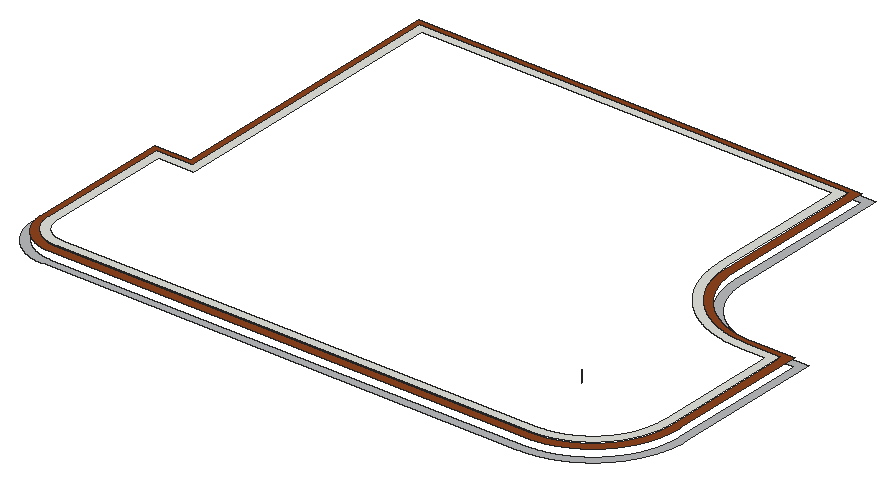
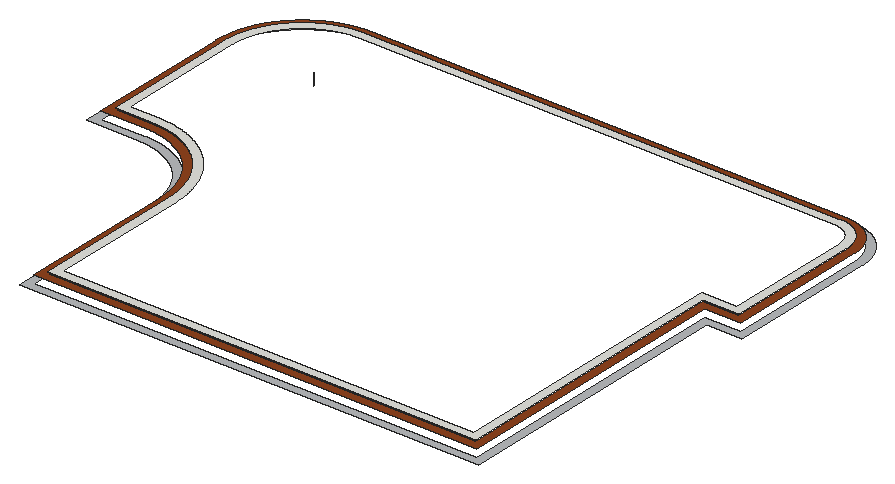
# SketchUp Ruby script. Lengths in inches.
U = 1.inch
M = Sketchup.active_model
def pt(a) = Geom::Point3d.new(a.map { |v| v * U })
def face(e, loops, mat)
  f = e.add_face(loops[0].map { |a| pt(a) })
  loops[1..].each { |l| e.add_face(l.map { |a| pt(a) }).erase! }
  f.material = f.back_material = mat if mat
  f
end
# faces: each face lists its corners as indices into pts; further lists are holes
def faces(e, pts, list, mat = nil) = list.each { |f| face(e, (f[0].is_a?(Array) ? f : [f]).map { |l| l.map { |i| pts[i] } }, mat) }
# xy, xz, yz: faces in a plane at the given z, y or x. An outline is a flat list of corners, or four numbers for a rectangle; further outlines are holes
def ring(l) = l.size == 4 ? [[l[0], l[1]], [l[2], l[1]], [l[2], l[3]], [l[0], l[3]]] : l.each_slice(2).to_a
def flat(e, list, mat, &to3) = list.each { |f| face(e, (f[0].is_a?(Array) ? f : [f]).map { |l| ring(l).map { |u, v| to3.(u, v) } }, mat) }
def xy(e, z, list, mat = nil) = flat(e, list, mat) { |x, y| [x, y, z] }
def xz(e, y, list, mat = nil) = flat(e, list, mat) { |x, z| [x, y, z] }
def yz(e, x, list, mat = nil) = flat(e, list, mat) { |y, z| [x, y, z] }
def lines(e, pts, list) = list.each { |a, b| e.add_line(pt(pts[a]), pt(pts[b])) }
# prism: a flat outline (further loops are holes) pulled along v
def prism(e, loops, v, mat = nil)
  f = face(e, loops, mat); d = Geom::Vector3d.new(v.map { |x| x * U })
  f.pushpull(f.normal.samedirection?(d) ? d.length : -d.length)
end
def box(e, o, s, mat = nil) = prism(e, [[o, [o[0] + s[0], o[1], o[2]], [o[0] + s[0], o[1] + s[1], o[2]], [o[0], o[1] + s[1], o[2]]]], [0, 0, s[2]], mat)
def at(x, y, z, deg = 0) = Geom::Transformation.translation(pt([x, y, z])) * Geom::Transformation.rotation(ORIGIN, Z_AXIS, deg.degrees)
def axes(o, x, y, z) = Geom::Transformation.new([*x, 0, *y, 0, *z, 0, *pt(o).to_a, 1])
def part(name) = M.definitions.add(name)
# library, detail: a bought-in or finely detailed component or shape, given as its bounding box
def library(name, o, s) = part(name).tap { |d| box(d.entities, o, s) }
def detail(e, o, s) = box(e.add_group.entities, o, s)
def put(e, d, t, mat = nil) = e.add_instance(d, t).tap { |i| i.material = mat if mat }
def group(e, t, mat = nil) = e.add_group.tap { |g| g.transformation = t; g.material = mat if mat }.entities
root = M.entities
M.materials.add("1427 AP 686 ARMOUR-N").color = [184, 186, 189]
M.materials.add("[Wood Fence]").color = [142, 67, 30]
xy(root,240,[[[20.991,129.924,20.843,129.925,20.686,129.928,20.529,129.934,20.372,129.941,20.215,129.95,20.059,129.961,19.902,129.975,19.746,129.99,19.59,130.008,19.434,130.027,19.278,130.049,19.123,130.072,18.968,130.098,18.813,130.125,18.659,130.155,18.505,130.187,18.352,130.22,18.199,130.256,18.046,130.294,17.894,130.333,17.743,130.375,17.592,130.419,17.442,130.464,17.292,130.512,17.143,130.561,16.994,130.613,16.847,130.666,16.7,130.721,16.553,130.779,16.408,130.838,16.263,130.899,16.119,130.962,15.976,131.027,15.834,131.093,15.693,131.162,15.552,131.232,15.413,131.305,15.274,131.379,15.137,131.454,15,131.532,14.865,131.611,14.73,131.693,14.597,131.776,14.464,131.86,14.333,131.947,14.203,132.035,14.074,132.125,13.947,132.216,13.82,132.309,13.695,132.404,13.571,132.501,13.448,132.599,13.327,132.698,13.207,132.799,13.088,132.902,12.854,133.112,12.74,133.22,12.627,133.329,12.515,133.439,12.404,133.551,12.296,133.664,12.188,133.779,12.082,133.895,11.978,134.012,11.875,134.131,11.774,134.251,11.674,134.373,11.576,134.495,11.48,134.619,11.385,134.744,11.292,134.871,11.2,134.999,11.111,135.127,11.022,135.258,10.936,135.389,10.851,135.521,10.768,135.654,10.687,135.789,10.608,135.924,10.53,136.061,10.454,136.198,10.38,136.337,10.308,136.476,10.238,136.617,10.169,136.758,10.102,136.9,10.038,137.044,9.975,137.1875,9.914,137.332,9.854,137.478,9.797,137.624,9.742,137.771,9.688,137.919,9.637,138.067,9.587,138.216,9.54,138.366,9.494,138.516,9.451,138.667,9.409,138.819,9.369,138.971,9.332,139.123,9.296,139.276,9.262,139.429,9.231,139.583,9.201,139.738,9.173,139.892,9.148,140.047,9.124,140.202,9.103,140.358,9.083,140.514,9.066,140.67,9.05,140.826,9.037,140.983,9.026,141.14,9.017,141.296,9.009,141.453,9.004,141.61,9.001,141.767,9,141.924,9,180,18,180,18,252,134,252,134,209.973,134.001,209.783,134.005,209.565,134.012,209.348,134.021,209.13,134.033,208.913,134.047,208.696,134.064,208.479,134.084,208.263,134.106,208.046,134.131,207.83,134.159,207.615,134.189,207.399,134.221,207.184,134.257,206.97,134.295,206.755,134.335,206.542,134.378,206.329,134.424,206.116,134.472,205.904,134.523,205.692,134.576,205.481,134.632,205.271,134.69,205.062,134.751,204.853,134.815,204.645,134.881,204.4375,134.949,204.231,135.02,204.026,135.094,203.821,135.17,203.617,135.248,203.414,135.329,203.212,135.412,203.011,135.498,202.811,135.586,202.613,135.676,202.415,135.769,202.218,135.864,202.022,135.962,201.828,136.062,201.635,136.164,201.443,136.268,201.252,136.375,201.063,136.484,200.875,136.596,200.688,136.709,200.502,136.825,200.318,136.943,200.136,137.064,199.954,137.186,199.775,137.311,199.596,137.4375,199.42,137.566,199.245,137.697,199.071,137.831,198.899,137.966,198.729,138.103,198.56,138.242,198.393,138.383,198.227,138.527,198.064,138.672,197.902,138.819,197.742,138.968,197.583,139.119,197.427,139.272,197.272,139.427,197.119,139.583,196.968,139.742,196.819,139.902,196.672,140.064,196.527,140.227,196.383,140.393,196.242,140.56,196.103,140.729,195.966,140.899,195.831,141.071,195.697,141.245,195.566,141.42,195.4375,141.596,195.311,141.775,195.186,141.954,195.064,142.136,194.943,142.318,194.825,142.502,194.709,142.688,194.596,142.875,194.484,143.063,194.375,143.252,194.268,143.443,194.164,143.635,194.062,143.828,193.962,144.022,193.864,144.218,193.769,144.415,193.676,144.613,193.586,144.811,193.498,145.011,193.412,145.212,193.329,145.414,193.248,145.617,193.17,145.821,193.094,146.026,193.02,146.231,192.949,146.4375,192.881,146.645,192.815,146.853,192.751,147.062,192.69,147.271,192.632,147.481,192.576,147.692,192.523,147.904,192.472,148.116,192.424,148.329,192.378,148.542,192.335,148.755,192.295,148.97,192.257,149.184,192.221,149.399,192.189,149.615,192.159,149.83,192.131,150.046,192.106,150.263,192.084,150.479,192.064,150.696,192.047,150.913,192.033,151.13,192.021,151.348,192.012,151.565,192.005,151.783,192.001,151.973,192,165,192,165,153.924,164.998,153.634,164.993,153.344,164.984,153.055,164.972,152.765,164.956,152.475,164.937,152.186,164.914,151.897,164.888,151.608,164.858,151.32,164.825,151.031,164.788,150.744,164.748,150.457,164.704,150.17,164.657,149.884,164.607,149.598,164.553,149.313,164.495,149.029,164.434,148.745,164.37,148.463,164.302,148.181,164.231,147.9,164.157,147.619,164.079,147.34,163.997,147.062,163.913,146.784,163.825,146.508,163.734,146.233,163.639,145.958,163.541,145.686,163.44,145.414,163.335,145.143,163.228,144.874,163.117,144.606,163.002,144.34,162.885,144.074,162.764,143.811,162.641,143.548,162.514,143.288,162.383,143.028,162.25,142.771,162.114,142.515,161.974,142.261,161.832,142.008,161.687,141.757,161.538,141.508,161.386,141.261,161.232,141.015,161.074,140.772,160.914,140.53,160.751,140.291,160.585,140.053,160.416,139.817,160.244,139.584,160.069,139.352,159.891,139.123,159.711,138.896,159.528,138.671,159.343,138.448,159.154,138.228,158.963,138.009,158.77,137.793,158.573,137.58,158.375,137.369,158.173,137.16,157.97,136.954,157.763,136.75,157.554,136.549,157.343,136.35,157.13,136.154,156.914,135.96,156.696,135.769,156.475,135.581,156.252,135.395,156.027,135.212,155.8,135.032,155.571,134.854,155.339,134.68,155.106,134.508,154.87,134.339,154.632,134.173,154.393,134.009,154.151,133.849,153.908,133.692,153.662,133.537,153.415,133.386,153.166,133.237,152.915,133.092,152.662,132.949,152.408,132.81,152.152,132.673,151.894,132.54,151.635,132.41,151.375,132.283,151.112,132.159,150.849,132.039,150.583,131.921,150.317,131.807,150.049,131.696,149.78,131.588,149.509,131.484,149.237,131.383,148.964,131.285,148.69,131.19,148.415,131.099,148.139,131.011,147.861,130.926,147.583,130.845,147.304,130.767,147.023,130.693,146.742,130.622,146.46,130.554,146.177,130.49,145.894,130.429,145.61,130.372,145.325,130.318,145.039,130.267,144.753,130.22,144.466,130.176,144.179,130.136,143.891,130.099,143.603,130.066,143.315,130.036,143.026,130.01,142.737,129.987,142.447,129.968,142.158,129.952,141.868,129.94,141.578,129.931,141.288,129.926,141.003,129.924],[21.005,131.924,140.992,131.924,141.264,131.926,141.53,131.931,141.796,131.939,142.061,131.95,142.327,131.965,142.592,131.982,142.857,132.003,143.122,132.027,143.386,132.054,143.65,132.085,143.914,132.118,144.177,132.155,144.44,132.195,144.702,132.238,144.964,132.285,145.225,132.334,145.486,132.387,145.746,132.443,146.005,132.502,146.263,132.564,146.521,132.629,146.778,132.697,147.034,132.769,147.289,132.843,147.544,132.921,147.797,133.001,148.049,133.085,148.301,133.172,148.551,133.261,148.8,133.354,149.048,133.45,149.295,133.549,149.54,133.65,149.785,133.755,150.028,133.863,150.269,133.973,150.51,134.087,150.749,134.203,150.986,134.322,151.223,134.444,151.457,134.569,151.69,134.697,151.922,134.828,152.152,134.961,152.38,135.097,152.607,135.236,152.832,135.378,153.055,135.522,153.277,135.669,153.496,135.819,153.714,135.971,153.93,136.126,154.144,136.284,154.356,136.444,154.567,136.606,154.775,136.772,154.981,136.939,155.185,137.109,155.388,137.282,155.588,137.457,155.786,137.635,155.981,137.814,156.175,137.997,156.366,138.181,156.555,138.368,156.742,138.557,156.927,138.748,157.109,138.942,157.289,139.138,157.466,139.336,157.641,139.536,157.814,139.738,157.984,139.942,158.152,140.148,158.317,140.357,158.48,140.567,158.64,140.779,158.798,140.993,158.952,141.209,159.105,141.427,159.255,141.647,159.402,141.868,159.546,142.091,159.6875,142.316,159.826,142.543,159.963,142.771,160.096,143.001,160.227,143.233,160.354,143.466,160.479,143.7,160.601,143.937,160.721,144.174,160.837,144.413,160.951,144.654,161.061,144.895,161.169,145.138,161.274,145.383,161.375,145.628,161.474,145.875,161.57,146.123,161.663,146.372,161.752,146.622,161.839,146.874,161.923,147.126,162.003,147.379,162.081,147.634,162.155,147.889,162.227,148.145,162.295,148.402,162.36,148.659,162.422,148.918,162.481,149.177,162.537,149.437,162.59,149.698,162.639,149.959,162.686,150.221,162.729,150.483,162.769,150.746,162.806,151.009,162.839,151.273,162.87,151.537,162.897,151.801,162.921,152.066,162.942,152.331,162.96,152.596,162.974,152.862,162.985,153.127,162.994,153.393,162.998,153.659,163,153.931,163,190,151.967,190,151.758,190.001,151.517,190.006,151.275,190.013,151.034,190.023,150.792,190.036,150.551,190.052,150.31,190.071,150.07,190.093,149.829,190.118,149.589,190.146,149.35,190.176,149.11,190.21,148.871,190.246,148.633,190.285,148.395,190.327,148.157,190.372,147.921,190.42,147.684,190.471,147.449,190.525,147.214,190.581,146.979,190.64,146.746,190.702,146.513,190.767,146.281,190.835,146.05,190.905,145.82,190.979,145.59,191.055,145.362,191.134,145.134,191.215,144.908,191.299,144.682,191.387,144.458,191.476,144.235,191.569,144.013,191.664,143.792,191.762,143.572,191.862,143.353,191.965,143.136,192.071,142.92,192.18,142.705,192.291,142.492,192.404,142.28,192.52,142.07,192.639,141.861,192.76,141.653,192.884,141.447,193.01,141.243,193.139,141.04,193.27,140.838,193.404,140.639,193.54,140.441,193.679,140.244,193.819,140.05,193.963,139.857,194.108,139.665,194.256,139.476,194.406,139.289,194.559,139.103,194.714,138.919,194.87,138.737,195.03,138.557,195.191,138.38,195.354,138.204,195.52,138.03,195.688,137.858,195.858,137.688,196.03,137.52,196.204,137.354,196.38,137.191,196.557,137.03,196.737,136.87,196.919,136.714,197.103,136.559,197.289,136.406,197.476,136.256,197.665,136.108,197.857,135.963,198.05,135.819,198.244,135.679,198.441,135.54,198.639,135.404,198.838,135.27,199.04,135.139,199.243,135.01,199.447,134.884,199.653,134.76,199.861,134.639,200.07,134.52,200.28,134.404,200.492,134.291,200.705,134.18,200.92,134.071,201.136,133.965,201.353,133.862,201.572,133.762,201.792,133.664,202.013,133.569,202.235,133.476,202.458,133.387,202.682,133.299,202.908,133.215,203.134,133.134,203.362,133.055,203.59,132.979,203.82,132.905,204.05,132.835,204.281,132.767,204.513,132.702,204.746,132.64,204.979,132.581,205.214,132.525,205.449,132.471,205.684,132.42,205.921,132.372,206.157,132.327,206.395,132.285,206.633,132.246,206.871,132.21,207.11,132.176,207.35,132.146,207.589,132.118,207.829,132.093,208.07,132.071,208.31,132.052,208.551,132.036,208.792,132.023,209.034,132.013,209.275,132.006,209.517,132.001,209.758,132,209.967,132,250,20,250,20,178,11,178,11,141.931,11.001,141.793,11.004,141.663,11.008,141.532,11.014,141.401,11.022,141.27,11.031,141.14,11.042,141.009,11.055,140.879,11.069,140.749,11.086,140.619,11.104,140.489,11.123,140.36,11.145,140.231,11.168,140.102,11.192,139.973,11.219,139.845,11.247,139.717,11.276,139.59,11.308,139.463,11.341,139.336,11.376,139.21,11.412,139.084,11.45,138.959,11.49,138.834,11.531,138.71,11.574,138.586,11.618,138.463,11.664,138.341,11.712,138.219,11.761,138.098,11.812,137.977,11.865,137.857,11.919,137.738,11.974,137.619,12.031,137.501,12.09,137.384,12.15,137.268,12.212,137.153,12.275,137.038,12.34,136.924,12.406,136.811,12.474,136.699,12.543,136.588,12.613,136.478,12.685,136.369,12.759,136.26,12.834,136.153,12.91,136.047,12.988,135.941,13.067,135.837,13.147,135.733,13.229,135.631,13.312,135.53,13.396,135.43,13.482,135.331,13.569,135.233,13.657,135.136,13.746,135.041,13.837,134.946,13.929,134.853,14.022,134.761,14.212,134.581,14.309,134.493,14.407,134.406,14.506,134.32,14.606,134.236,14.707,134.153,14.809,134.071,14.913,133.991,15.017,133.912,15.122,133.834,15.229,133.758,15.336,133.683,15.444,133.61,15.554,133.538,15.664,133.467,15.775,133.398,15.887,133.33,16,133.264,16.114,133.199,16.229,133.136,16.344,133.075,16.46,133.014,16.577,132.956,16.695,132.899,16.814,132.843,16.933,132.789,17.053,132.736,17.173,132.686,17.295,132.636,17.416,132.589,17.539,132.542,17.662,132.498,17.786,132.455,17.91,132.414,18.035,132.374,18.16,132.336,18.286,132.3,18.412,132.265,18.539,132.232,18.666,132.201,18.793,132.171,18.921,132.143,19.049,132.117,19.178,132.092,19.307,132.069,19.436,132.048,19.565,132.028,19.695,132.01,19.825,131.994,19.955,131.979,20.085,131.966,20.216,131.955,20.346,131.946,20.477,131.938,20.607,131.932,20.738,131.928,20.869,131.925]]],"1427 AP 686 ARMOUR-N")
xy(root,242,[[[21.005,131.924,20.869,131.925,20.738,131.928,20.607,131.932,20.477,131.938,20.346,131.946,20.216,131.955,20.085,131.966,19.955,131.979,19.825,131.994,19.695,132.01,19.565,132.028,19.436,132.048,19.307,132.069,19.178,132.092,19.049,132.117,18.921,132.143,18.793,132.171,18.666,132.201,18.539,132.232,18.412,132.265,18.286,132.3,18.16,132.336,18.035,132.374,17.91,132.414,17.786,132.455,17.662,132.498,17.539,132.542,17.416,132.589,17.295,132.636,17.173,132.686,17.053,132.736,16.933,132.789,16.814,132.843,16.695,132.899,16.577,132.956,16.46,133.014,16.344,133.075,16.229,133.136,16.114,133.199,16,133.264,15.887,133.33,15.775,133.398,15.664,133.467,15.554,133.538,15.444,133.61,15.336,133.683,15.229,133.758,15.122,133.834,15.017,133.912,14.913,133.991,14.809,134.071,14.707,134.153,14.606,134.236,14.506,134.32,14.407,134.406,14.309,134.493,14.212,134.581,14.022,134.761,13.929,134.853,13.837,134.946,13.746,135.041,13.657,135.136,13.569,135.233,13.482,135.331,13.396,135.43,13.312,135.53,13.229,135.631,13.147,135.733,13.067,135.837,12.988,135.941,12.91,136.047,12.834,136.153,12.759,136.26,12.685,136.369,12.613,136.478,12.543,136.588,12.474,136.699,12.406,136.811,12.34,136.924,12.275,137.038,12.212,137.153,12.15,137.268,12.09,137.384,12.031,137.501,11.974,137.619,11.919,137.738,11.865,137.857,11.812,137.977,11.761,138.098,11.712,138.219,11.664,138.341,11.618,138.463,11.574,138.586,11.531,138.71,11.49,138.834,11.45,138.959,11.412,139.084,11.376,139.21,11.341,139.336,11.308,139.463,11.276,139.59,11.247,139.717,11.219,139.845,11.192,139.973,11.168,140.102,11.145,140.231,11.123,140.36,11.104,140.489,11.086,140.619,11.069,140.749,11.055,140.879,11.042,141.009,11.031,141.14,11.022,141.27,11.014,141.401,11.008,141.532,11.004,141.663,11.001,141.793,11,141.931,11,178,20,178,20,250,132,250,132,209.967,132.001,209.758,132.006,209.517,132.013,209.275,132.023,209.034,132.036,208.792,132.052,208.551,132.071,208.31,132.093,208.07,132.118,207.829,132.146,207.589,132.176,207.35,132.21,207.11,132.246,206.871,132.285,206.633,132.327,206.395,132.372,206.157,132.42,205.921,132.471,205.684,132.525,205.449,132.581,205.214,132.64,204.979,132.702,204.746,132.767,204.513,132.835,204.281,132.905,204.05,132.979,203.82,133.055,203.59,133.134,203.362,133.215,203.134,133.299,202.908,133.387,202.682,133.476,202.458,133.569,202.235,133.664,202.013,133.762,201.792,133.862,201.572,133.965,201.353,134.071,201.136,134.18,200.92,134.291,200.705,134.404,200.492,134.52,200.28,134.639,200.07,134.76,199.861,134.884,199.653,135.01,199.447,135.139,199.243,135.27,199.04,135.404,198.838,135.54,198.639,135.679,198.441,135.819,198.244,135.963,198.05,136.108,197.857,136.256,197.665,136.406,197.476,136.559,197.289,136.714,197.103,136.87,196.919,137.03,196.737,137.191,196.557,137.354,196.38,137.52,196.204,137.688,196.03,137.858,195.858,138.03,195.688,138.204,195.52,138.38,195.354,138.557,195.191,138.737,195.03,138.919,194.87,139.103,194.714,139.289,194.559,139.476,194.406,139.665,194.256,139.857,194.108,140.05,193.963,140.244,193.819,140.441,193.679,140.639,193.54,140.838,193.404,141.04,193.27,141.243,193.139,141.447,193.01,141.653,192.884,141.861,192.76,142.07,192.639,142.28,192.52,142.492,192.404,142.705,192.291,142.92,192.18,143.136,192.071,143.353,191.965,143.572,191.862,143.792,191.762,144.013,191.664,144.235,191.569,144.458,191.476,144.682,191.387,144.908,191.299,145.134,191.215,145.362,191.134,145.59,191.055,145.82,190.979,146.05,190.905,146.281,190.835,146.513,190.767,146.746,190.702,146.979,190.64,147.214,190.581,147.449,190.525,147.684,190.471,147.921,190.42,148.157,190.372,148.395,190.327,148.633,190.285,148.871,190.246,149.11,190.21,149.35,190.176,149.589,190.146,149.829,190.118,150.07,190.093,150.31,190.071,150.551,190.052,150.792,190.036,151.034,190.023,151.275,190.013,151.517,190.006,151.758,190.001,151.967,190,163,190,163,153.931,162.998,153.659,162.994,153.393,162.985,153.127,162.974,152.862,162.96,152.596,162.942,152.331,162.921,152.066,162.897,151.801,162.87,151.537,162.839,151.273,162.806,151.009,162.769,150.746,162.729,150.483,162.686,150.221,162.639,149.959,162.59,149.698,162.537,149.437,162.481,149.177,162.422,148.918,162.36,148.659,162.295,148.402,162.227,148.145,162.155,147.889,162.081,147.634,162.003,147.379,161.923,147.126,161.839,146.874,161.752,146.622,161.663,146.372,161.57,146.123,161.474,145.875,161.375,145.628,161.274,145.383,161.169,145.138,161.061,144.895,160.951,144.654,160.837,144.413,160.721,144.174,160.601,143.937,160.479,143.7,160.354,143.466,160.227,143.233,160.096,143.001,159.963,142.771,159.826,142.543,159.6875,142.316,159.546,142.091,159.402,141.868,159.255,141.647,159.105,141.427,158.952,141.209,158.798,140.993,158.64,140.779,158.48,140.567,158.317,140.357,158.152,140.148,157.984,139.942,157.814,139.738,157.641,139.536,157.466,139.336,157.289,139.138,157.109,138.942,156.927,138.748,156.742,138.557,156.555,138.368,156.366,138.181,156.175,137.997,155.981,137.814,155.786,137.635,155.588,137.457,155.388,137.282,155.185,137.109,154.981,136.939,154.775,136.772,154.567,136.606,154.356,136.444,154.144,136.284,153.93,136.126,153.714,135.971,153.496,135.819,153.277,135.669,153.055,135.522,152.832,135.378,152.607,135.236,152.38,135.097,152.152,134.961,151.922,134.828,151.69,134.697,151.457,134.569,151.223,134.444,150.986,134.322,150.749,134.203,150.51,134.087,150.269,133.973,150.028,133.863,149.785,133.755,149.54,133.65,149.295,133.549,149.048,133.45,148.8,133.354,148.551,133.261,148.301,133.172,148.049,133.085,147.797,133.001,147.544,132.921,147.289,132.843,147.034,132.769,146.778,132.697,146.521,132.629,146.263,132.564,146.005,132.502,145.746,132.443,145.486,132.387,145.225,132.334,144.964,132.285,144.702,132.238,144.44,132.195,144.177,132.155,143.914,132.118,143.65,132.085,143.386,132.054,143.122,132.027,142.857,132.003,142.592,131.982,142.327,131.965,142.061,131.95,141.796,131.939,141.53,131.931,141.264,131.926,140.992,131.924],[21.013,133.924,140.986,133.924,141.24,133.926,141.482,133.93,141.723,133.9375,141.965,133.948,142.206,133.961,142.447,133.977,142.688,133.996,142.929,134.018,143.169,134.043,143.409,134.07,143.649,134.101,143.888,134.134,144.127,134.171,144.366,134.21,144.604,134.252,144.841,134.297,145.078,134.345,145.314,134.396,145.55,134.449,145.785,134.506,146.019,134.565,146.253,134.627,146.485,134.692,146.717,134.76,146.949,134.83,147.179,134.903,147.408,134.979,147.637,135.058,147.864,135.14,148.091,135.224,148.316,135.311,148.541,135.401,148.764,135.493,148.986,135.589,149.207,135.686,149.427,135.787,149.645,135.89,149.863,135.996,150.079,136.104,150.293,136.215,150.506,136.329,150.718,136.445,150.929,136.564,151.138,136.685,151.346,136.809,151.552,136.935,151.756,137.064,151.959,137.195,152.16,137.329,152.36,137.465,152.558,137.603,152.755,137.744,152.949,137.887,153.142,138.033,153.333,138.181,153.523,138.331,153.71,138.483,153.896,138.638,154.08,138.795,154.261,138.954,154.441,139.116,154.619,139.279,154.795,139.445,154.969,139.612,155.141,139.782,155.311,139.954,155.479,140.128,155.644,140.304,155.808,140.482,155.969,140.662,156.128,140.844,156.285,141.028,156.44,141.213,156.593,141.401,156.743,141.59,156.891,141.781,157.036,141.974,157.179,142.169,157.32,142.365,157.459,142.563,157.595,142.763,157.729,142.964,157.86,143.167,157.989,143.372,158.115,143.578,158.239,143.785,158.36,143.994,158.479,144.205,158.595,144.417,158.708,144.63,158.819,144.845,158.928,145.061,159.034,145.278,159.137,145.496,159.237,145.716,159.335,145.937,159.43,146.159,159.523,146.383,159.613,146.607,159.7,146.832,159.784,147.059,159.866,147.286,159.945,147.515,160.021,147.744,160.094,147.974,160.164,148.206,160.232,148.4375,160.297,148.67,160.359,148.904,160.418,149.138,160.475,149.373,160.528,149.609,160.579,149.845,160.627,150.082,160.672,150.319,160.714,150.557,160.753,150.796,160.79,151.035,160.823,151.274,160.854,151.514,160.882,151.754,160.906,151.994,160.928,152.235,160.947,152.476,160.963,152.717,160.977,152.958,160.987,153.2,160.994,153.441,160.998,153.683,161,153.937,161,188,151.961,188,151.734,188.001,151.468,188.006,151.203,188.014,150.937,188.025,150.672,188.04,150.406,188.058,150.141,188.078,149.877,188.102,149.612,188.13,149.348,188.16,149.084,188.194,148.821,188.231,148.558,188.271,148.296,188.314,148.034,188.36,147.773,188.41,147.513,188.462,147.253,188.518,146.993,188.577,146.735,188.639,146.477,188.704,146.22,188.773,145.964,188.844,145.709,188.918,145.455,188.996,145.202,189.077,144.949,189.16,144.698,189.247,144.448,189.337,144.199,189.429,143.951,189.525,143.704,189.624,143.458,189.726,143.214,189.83,142.971,189.938,142.729,190.049,142.489,190.162,142.25,190.278,142.012,190.398,141.776,190.52,141.541,190.645,141.308,190.772,141.077,190.903,140.847,191.036,140.618,191.173,140.392,191.312,140.167,191.453,139.944,191.597,139.722,191.744,139.502,191.894,139.285,192.046,139.069,192.201,138.854,192.359,138.642,192.519,138.432,192.682,138.224,192.847,138.018,193.015,137.813,193.185,137.611,193.358,137.411,193.533,137.213,193.71,137.017,193.89,136.824,194.072,136.633,194.257,136.443,194.443,136.257,194.633,136.072,194.824,135.89,195.017,135.71,195.213,135.533,195.411,135.358,195.611,135.185,195.813,135.015,196.018,134.847,196.224,134.682,196.432,134.519,196.642,134.359,196.854,134.201,197.069,134.046,197.285,133.894,197.502,133.744,197.722,133.597,197.944,133.453,198.167,133.312,198.392,133.173,198.618,133.036,198.847,132.903,199.077,132.772,199.308,132.645,199.541,132.52,199.776,132.398,200.012,132.278,200.25,132.162,200.489,132.049,200.729,131.938,200.971,131.83,201.214,131.726,201.458,131.624,201.704,131.525,201.951,131.429,202.199,131.337,202.448,131.247,202.698,131.16,202.949,131.077,203.202,130.996,203.455,130.918,203.709,130.844,203.964,130.773,204.22,130.704,204.477,130.639,204.735,130.577,204.993,130.518,205.253,130.462,205.513,130.41,205.773,130.36,206.034,130.314,206.296,130.271,206.558,130.231,206.821,130.194,207.084,130.16,207.348,130.13,207.612,130.102,207.877,130.078,208.141,130.058,208.406,130.04,208.672,130.025,208.937,130.014,209.203,130.006,209.468,130.001,209.734,130,209.961,130,248,22,248,22,176,13,176,13,141.9375,13.001,141.82,13.003,141.715,13.006,141.61,13.011,141.506,13.017,141.401,13.025,141.297,13.034,141.192,13.044,141.088,13.056,140.984,13.069,140.88,13.083,140.776,13.099,140.673,13.116,140.57,13.134,140.466,13.154,140.364,13.175,140.261,13.197,140.159,13.221,140.057,13.246,139.955,13.273,139.854,13.301,139.753,13.33,139.652,13.36,139.552,13.392,139.452,13.425,139.353,13.459,139.254,13.495,139.155,13.532,139.057,13.57,138.96,13.609,138.863,13.65,138.766,13.692,138.671,13.735,138.575,13.779,138.48,13.825,138.386,13.872,138.292,13.92,138.199,14.02,138.015,14.072,137.924,14.125,137.834,14.179,137.744,14.234,137.655,14.291,137.567,14.348,137.48,14.407,137.393,14.467,137.307,14.528,137.222,14.59,137.138,14.653,137.054,14.783,136.89,14.849,136.809,14.917,136.729,14.985,136.65,15.055,136.571,15.126,136.494,15.197,136.418,15.27,136.342,15.343,136.268,15.418,136.194,15.493,136.121,15.647,135.979,15.725,135.91,15.805,135.841,15.885,135.774,15.966,135.707,16.047,135.642,16.13,135.578,16.214,135.514,16.298,135.452,16.383,135.391,16.469,135.331,16.643,135.215,16.731,135.159,16.82,135.103,16.91,135.049,17,134.996,17.091,134.944,17.183,134.894,17.275,134.845,17.368,134.796,17.462,134.749,17.556,134.704,17.651,134.659,17.746,134.616,17.842,134.574,17.939,134.533,18.036,134.494,18.133,134.456,18.231,134.419,18.33,134.383,18.429,134.349,18.528,134.316,18.628,134.284,18.728,134.254,18.829,134.225,18.93,134.197,19.031,134.171,19.133,134.145,19.337,134.099,19.439,134.078,19.542,134.058,19.645,134.04,19.749,134.023,19.852,134.007,19.956,133.993,20.06,133.98,20.164,133.968,20.268,133.958,20.372,133.949,20.477,133.942,20.581,133.935,20.791,133.927,20.895,133.925]]],"[Wood Fence]")
xy(root,242.5,[[[21.013,133.924,20.895,133.925,20.791,133.927,20.581,133.935,20.477,133.942,20.372,133.949,20.268,133.958,20.164,133.968,20.06,133.98,19.956,133.993,19.852,134.007,19.749,134.023,19.645,134.04,19.542,134.058,19.439,134.078,19.337,134.099,19.133,134.145,19.031,134.171,18.93,134.197,18.829,134.225,18.728,134.254,18.628,134.284,18.528,134.316,18.429,134.349,18.33,134.383,18.231,134.419,18.133,134.456,18.036,134.494,17.939,134.533,17.842,134.574,17.746,134.616,17.651,134.659,17.556,134.704,17.462,134.749,17.368,134.796,17.275,134.845,17.183,134.894,17.091,134.944,17,134.996,16.91,135.049,16.82,135.103,16.731,135.159,16.643,135.215,16.469,135.331,16.383,135.391,16.298,135.452,16.214,135.514,16.13,135.578,16.047,135.642,15.966,135.707,15.885,135.774,15.805,135.841,15.725,135.91,15.647,135.979,15.493,136.121,15.418,136.194,15.343,136.268,15.27,136.342,15.197,136.418,15.126,136.494,15.055,136.571,14.985,136.65,14.917,136.729,14.849,136.809,14.783,136.89,14.653,137.054,14.59,137.138,14.528,137.222,14.467,137.307,14.407,137.393,14.348,137.48,14.291,137.567,14.234,137.655,14.179,137.744,14.125,137.834,14.072,137.924,14.02,138.015,13.92,138.199,13.872,138.292,13.825,138.386,13.779,138.48,13.735,138.575,13.692,138.671,13.65,138.766,13.609,138.863,13.57,138.96,13.532,139.057,13.495,139.155,13.459,139.254,13.425,139.353,13.392,139.452,13.36,139.552,13.33,139.652,13.301,139.753,13.273,139.854,13.246,139.955,13.221,140.057,13.197,140.159,13.175,140.261,13.154,140.364,13.134,140.466,13.116,140.57,13.099,140.673,13.083,140.776,13.069,140.88,13.056,140.984,13.044,141.088,13.034,141.192,13.025,141.297,13.017,141.401,13.011,141.506,13.006,141.61,13.003,141.715,13.001,141.82,13,141.9375,13,176,22,176,22,248,130,248,130,209.961,130.001,209.734,130.006,209.468,130.014,209.203,130.025,208.937,130.04,208.672,130.058,208.406,130.078,208.141,130.102,207.877,130.13,207.612,130.16,207.348,130.194,207.084,130.231,206.821,130.271,206.558,130.314,206.296,130.36,206.034,130.41,205.773,130.462,205.513,130.518,205.253,130.577,204.993,130.639,204.735,130.704,204.477,130.773,204.22,130.844,203.964,130.918,203.709,130.996,203.455,131.077,203.202,131.16,202.949,131.247,202.698,131.337,202.448,131.429,202.199,131.525,201.951,131.624,201.704,131.726,201.458,131.83,201.214,131.938,200.971,132.049,200.729,132.162,200.489,132.278,200.25,132.398,200.012,132.52,199.776,132.645,199.541,132.772,199.308,132.903,199.077,133.036,198.847,133.173,198.618,133.312,198.392,133.453,198.167,133.597,197.944,133.744,197.722,133.894,197.502,134.046,197.285,134.201,197.069,134.359,196.854,134.519,196.642,134.682,196.432,134.847,196.224,135.015,196.018,135.185,195.813,135.358,195.611,135.533,195.411,135.71,195.213,135.89,195.017,136.072,194.824,136.257,194.633,136.443,194.443,136.633,194.257,136.824,194.072,137.017,193.89,137.213,193.71,137.411,193.533,137.611,193.358,137.813,193.185,138.018,193.015,138.224,192.847,138.432,192.682,138.642,192.519,138.854,192.359,139.069,192.201,139.285,192.046,139.502,191.894,139.722,191.744,139.944,191.597,140.167,191.453,140.392,191.312,140.618,191.173,140.847,191.036,141.077,190.903,141.308,190.772,141.541,190.645,141.776,190.52,142.012,190.398,142.25,190.278,142.489,190.162,142.729,190.049,142.971,189.938,143.214,189.83,143.458,189.726,143.704,189.624,143.951,189.525,144.199,189.429,144.448,189.337,144.698,189.247,144.949,189.16,145.202,189.077,145.455,188.996,145.709,188.918,145.964,188.844,146.22,188.773,146.477,188.704,146.735,188.639,146.993,188.577,147.253,188.518,147.513,188.462,147.773,188.41,148.034,188.36,148.296,188.314,148.558,188.271,148.821,188.231,149.084,188.194,149.348,188.16,149.612,188.13,149.877,188.102,150.141,188.078,150.406,188.058,150.672,188.04,150.937,188.025,151.203,188.014,151.468,188.006,151.734,188.001,151.961,188,161,188,161,153.937,160.998,153.683,160.994,153.441,160.987,153.2,160.977,152.958,160.963,152.717,160.947,152.476,160.928,152.235,160.906,151.994,160.882,151.754,160.854,151.514,160.823,151.274,160.79,151.035,160.753,150.796,160.714,150.557,160.672,150.319,160.627,150.082,160.579,149.845,160.528,149.609,160.475,149.373,160.418,149.138,160.359,148.904,160.297,148.67,160.232,148.4375,160.164,148.206,160.094,147.974,160.021,147.744,159.945,147.515,159.866,147.286,159.784,147.059,159.7,146.832,159.613,146.607,159.523,146.383,159.43,146.159,159.335,145.937,159.237,145.716,159.137,145.496,159.034,145.278,158.928,145.061,158.819,144.845,158.708,144.63,158.595,144.417,158.479,144.205,158.36,143.994,158.239,143.785,158.115,143.578,157.989,143.372,157.86,143.167,157.729,142.964,157.595,142.763,157.459,142.563,157.32,142.365,157.179,142.169,157.036,141.974,156.891,141.781,156.743,141.59,156.593,141.401,156.44,141.213,156.285,141.028,156.128,140.844,155.969,140.662,155.808,140.482,155.644,140.304,155.479,140.128,155.311,139.954,155.141,139.782,154.969,139.612,154.795,139.445,154.619,139.279,154.441,139.116,154.261,138.954,154.08,138.795,153.896,138.638,153.71,138.483,153.523,138.331,153.333,138.181,153.142,138.033,152.949,137.887,152.755,137.744,152.558,137.603,152.36,137.465,152.16,137.329,151.959,137.195,151.756,137.064,151.552,136.935,151.346,136.809,151.138,136.685,150.929,136.564,150.718,136.445,150.506,136.329,150.293,136.215,150.079,136.104,149.863,135.996,149.645,135.89,149.427,135.787,149.207,135.686,148.986,135.589,148.764,135.493,148.541,135.401,148.316,135.311,148.091,135.224,147.864,135.14,147.637,135.058,147.408,134.979,147.179,134.903,146.949,134.83,146.717,134.76,146.485,134.692,146.253,134.627,146.019,134.565,145.785,134.506,145.55,134.449,145.314,134.396,145.078,134.345,144.841,134.297,144.604,134.252,144.366,134.21,144.127,134.171,143.888,134.134,143.649,134.101,143.409,134.07,143.169,134.043,142.929,134.018,142.688,133.996,142.447,133.977,142.206,133.961,141.965,133.948,141.723,133.9375,141.482,133.93,141.24,133.926,140.986,133.924],[21.02,135.924,140.98,135.924,141.216,135.926,141.433,135.93,141.651,135.936,141.868,135.946,142.085,135.957,142.302,135.972,142.519,135.989,142.736,136.009,142.952,136.031,143.168,136.056,143.384,136.083,143.599,136.113,143.814,136.146,144.029,136.181,144.243,136.219,144.457,136.26,144.67,136.303,144.883,136.349,145.095,136.397,145.306,136.448,145.517,136.501,145.727,136.557,145.937,136.615,146.146,136.676,146.354,136.74,146.561,136.805,146.767,136.874,146.973,136.945,147.178,137.018,147.382,137.094,147.584,137.173,147.786,137.253,147.987,137.337,148.187,137.422,148.386,137.51,148.584,137.601,148.781,137.694,148.976,137.789,149.171,137.886,149.364,137.986,149.556,138.089,149.746,138.193,149.936,138.3,150.124,138.409,150.311,138.52,150.496,138.634,150.68,138.75,150.863,138.868,151.044,138.988,151.224,139.111,151.402,139.235,151.579,139.362,151.754,139.491,151.928,139.622,152.1,139.755,152.27,139.89,152.439,140.028,152.606,140.167,152.771,140.308,152.935,140.451,153.097,140.597,153.257,140.744,153.416,140.893,153.572,141.044,153.727,141.197,153.88,141.351,154.031,141.508,154.18,141.666,154.327,141.826,154.472,141.988,154.616,142.152,154.757,142.317,154.896,142.484,155.033,142.653,155.168,142.824,155.302,142.996,155.433,143.169,155.561,143.344,155.688,143.521,155.813,143.699,155.935,143.879,156.056,144.06,156.174,144.243,156.29,144.427,156.403,144.612,156.515,144.799,156.624,144.987,156.731,145.177,156.835,145.368,156.9375,145.56,157.037,145.753,157.135,145.947,157.23,146.143,157.323,146.339,157.414,146.537,157.502,146.736,157.587,146.936,157.671,147.137,157.751,147.339,157.83,147.542,157.906,147.746,157.979,147.95,158.05,148.156,158.119,148.362,158.185,148.57,158.248,148.778,158.309,148.986,158.367,149.196,158.423,149.406,158.477,149.617,158.527,149.828,158.576,150.041,158.621,150.253,158.664,150.466,158.705,150.68,158.743,150.894,158.778,151.109,158.811,151.324,158.841,151.539,158.869,151.755,158.893,151.971,158.916,152.1875,158.935,152.404,158.953,152.621,158.967,152.838,158.979,153.055,158.988,153.272,158.995,153.49,158.999,153.707,159,153.943,159,186,151.955,186,151.71,186.001,151.42,186.007,151.13,186.015,150.84,186.028,150.551,186.044,150.262,186.063,149.972,186.086,149.684,186.112,149.395,186.142,149.107,186.175,148.819,186.211,148.532,186.252,148.246,186.295,147.959,186.342,147.674,186.393,147.389,186.447,147.105,186.504,146.821,186.565,146.538,186.629,146.256,186.697,145.975,186.768,145.695,186.843,145.416,186.921,145.137,187.002,144.86,187.086,144.584,187.174,144.308,187.266,144.034,187.36,143.761,187.458,143.489,187.559,143.219,187.664,142.95,187.772,142.682,187.883,142.415,187.997,142.15,188.114,141.886,188.235,141.624,188.359,141.363,188.486,141.104,188.616,140.847,188.749,140.591,188.885,140.336,189.025,140.084,189.167,139.833,189.3125,139.584,189.461,139.336,189.613,139.091,189.767,138.848,189.924,138.606,190.085,138.366,190.248,138.129,190.414,137.893,190.583,137.659,190.755,137.428,190.93,137.199,191.107,136.971,191.288,136.746,191.471,136.524,191.656,136.303,191.845,136.085,192.036,135.869,192.229,135.655,192.425,135.444,192.624,135.236,192.825,135.029,193.029,134.825,193.236,134.624,193.444,134.425,193.655,134.229,193.869,134.036,194.085,133.845,194.303,133.656,194.524,133.471,194.746,133.288,194.971,133.107,195.199,132.93,195.428,132.755,195.659,132.583,195.893,132.414,196.129,132.248,196.366,132.085,196.606,131.924,196.848,131.767,197.091,131.613,197.336,131.461,197.584,131.3125,197.833,131.167,198.084,131.025,198.336,130.885,198.591,130.749,198.847,130.616,199.104,130.486,199.363,130.359,199.624,130.235,199.886,130.114,200.15,129.997,200.415,129.883,200.682,129.772,200.95,129.664,201.219,129.559,201.489,129.458,201.761,129.36,202.034,129.266,202.308,129.174,202.584,129.086,202.86,129.002,203.137,128.921,203.416,128.843,203.695,128.768,203.975,128.697,204.256,128.629,204.538,128.565,204.821,128.504,205.105,128.447,205.389,128.393,205.674,128.342,205.959,128.295,206.246,128.252,206.532,128.211,206.819,128.175,207.107,128.142,207.395,128.112,207.684,128.086,207.972,128.063,208.262,128.044,208.551,128.028,208.84,128.015,209.13,128.007,209.42,128.001,209.71,128,209.955,128,246,24,246,24,174,15,174,15,141.944,15.001,141.846,15.002,141.767,15.005,141.689,15.008,141.61,15.013,141.532,15.019,141.454,15.025,141.375,15.033,141.297,15.042,141.219,15.052,141.141,15.0625,141.063,15.074,140.986,15.087,140.908,15.101,140.831,15.131,140.677,15.148,140.6,15.166,140.524,15.185,140.447,15.205,140.371,15.225,140.296,15.247,140.22,15.27,140.145,15.294,140.07,15.344,139.922,15.371,139.848,15.399,139.774,15.427,139.701,15.457,139.628,15.487,139.556,15.551,139.412,15.585,139.341,15.619,139.271,15.654,139.2,15.69,139.131,15.727,139.061,15.765,138.993,15.804,138.924,15.844,138.857,15.884,138.789,15.968,138.657,16.011,138.591,16.055,138.526,16.1,138.462,16.146,138.398,16.193,138.334,16.24,138.272,16.288,138.21,16.337,138.149,16.387,138.088,16.489,137.968,16.541,137.91,16.594,137.852,16.648,137.794,16.702,137.738,16.813,137.627,16.87,137.572,16.927,137.519,16.985,137.466,17.044,137.413,17.103,137.362,17.164,137.311,17.224,137.262,17.348,137.164,17.41,137.117,17.473,137.07,17.537,137.025,17.602,136.98,17.732,136.892,17.798,136.85,17.932,136.768,18,136.728,18.068,136.69,18.137,136.652,18.206,136.615,18.276,136.578,18.346,136.543,18.417,136.509,18.488,136.476,18.56,136.443,18.704,136.381,18.85,136.323,18.923,136.295,19.071,136.243,19.146,136.218,19.221,136.194,19.371,136.15,19.447,136.129,19.523,136.109,19.599,136.09,19.676,136.072,19.83,136.04,19.907,136.025,19.984,136.011,20.062,135.998,20.139,135.987,20.217,135.976,20.295,135.966,20.373,135.957,20.529,135.943,20.608,135.9375,20.686,135.933,20.765,135.929,20.843,135.927,20.922,135.925]]])
p = [[136.5,155.924,242],[136.501,156.003,242],[136.501,156.003,245],[136.5,155.924,245]]
faces(root,p,[[0,1,2,3]])
